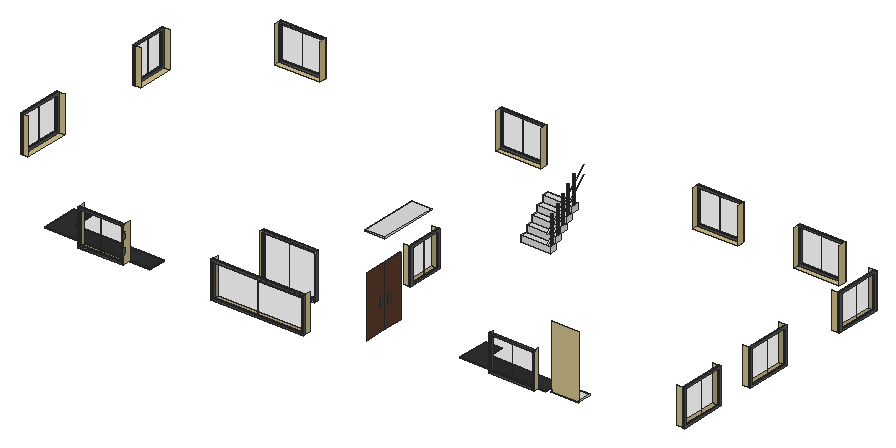
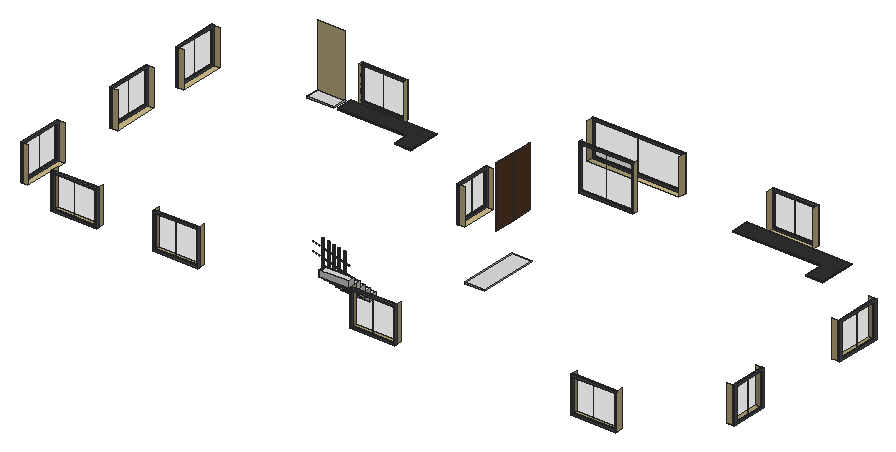
# SketchUp Ruby script. Lengths in inches.
U = 1.inch
M = Sketchup.active_model
def pt(a) = Geom::Point3d.new(a.map { |v| v * U })
def face(e, loops, mat)
  f = e.add_face(loops[0].map { |a| pt(a) })
  loops[1..].each { |l| e.add_face(l.map { |a| pt(a) }).erase! }
  f.material = f.back_material = mat if mat
  f
end
# faces: each face lists its corners as indices into pts; further lists are holes
def faces(e, pts, list, mat = nil) = list.each { |f| face(e, (f[0].is_a?(Array) ? f : [f]).map { |l| l.map { |i| pts[i] } }, mat) }
# xy, xz, yz: faces in a plane at the given z, y or x. An outline is a flat list of corners, or four numbers for a rectangle; further outlines are holes
def ring(l) = l.size == 4 ? [[l[0], l[1]], [l[2], l[1]], [l[2], l[3]], [l[0], l[3]]] : l.each_slice(2).to_a
def flat(e, list, mat, &to3) = list.each { |f| face(e, (f[0].is_a?(Array) ? f : [f]).map { |l| ring(l).map { |u, v| to3.(u, v) } }, mat) }
def xy(e, z, list, mat = nil) = flat(e, list, mat) { |x, y| [x, y, z] }
def xz(e, y, list, mat = nil) = flat(e, list, mat) { |x, z| [x, y, z] }
def yz(e, x, list, mat = nil) = flat(e, list, mat) { |y, z| [x, y, z] }
def lines(e, pts, list) = list.each { |a, b| e.add_line(pt(pts[a]), pt(pts[b])) }
# prism: a flat outline (further loops are holes) pulled along v
def prism(e, loops, v, mat = nil)
  f = face(e, loops, mat); d = Geom::Vector3d.new(v.map { |x| x * U })
  f.pushpull(f.normal.samedirection?(d) ? d.length : -d.length)
end
def box(e, o, s, mat = nil) = prism(e, [[o, [o[0] + s[0], o[1], o[2]], [o[0] + s[0], o[1] + s[1], o[2]], [o[0], o[1] + s[1], o[2]]]], [0, 0, s[2]], mat)
def at(x, y, z, deg = 0) = Geom::Transformation.translation(pt([x, y, z])) * Geom::Transformation.rotation(ORIGIN, Z_AXIS, deg.degrees)
def axes(o, x, y, z) = Geom::Transformation.new([*x, 0, *y, 0, *z, 0, *pt(o).to_a, 1])
def part(name) = M.definitions.add(name)
# library, detail: a bought-in or finely detailed component or shape, given as its bounding box
def library(name, o, s) = part(name).tap { |d| box(d.entities, o, s) }
def detail(e, o, s) = box(e.add_group.entities, o, s)
def put(e, d, t, mat = nil) = e.add_instance(d, t).tap { |i| i.material = mat if mat }
def group(e, t, mat = nil) = e.add_group.tap { |g| g.transformation = t; g.material = mat if mat }.entities
root = M.entities
M.materials.add("Flooring Laminate Dark Smoked 375cm").color = [91, 60, 43]
M.materials.add("Glass Smoked Distorted 001").color = [38, 38, 38]
M.materials["Glass Smoked Distorted 001"].alpha = 0.1
M.materials.add("Granite Black Pearl 150cm").color = [48, 48, 48]
M.materials.add("Marble White SSS 100cm").color = [222, 222, 222]
M.materials.add("Metal Sandblasted Black 200cm").color = [86, 90, 95]
M.materials.add("Wall Paint Fine Grain 01 Yellow 100cm").color = [207, 190, 139]
c1 = part("Group\#124")
p = [[0,61.03,56],[0.26,0,0],[0.46,0,0],[0.2,61.03,56]]
faces(c1.entities,p,[[0,1,2,3]])
c2 = part("Group\#8")
box(c2.entities,[0,0,0],[59.16,0.31,44])
c3 = part("Group\#10")
box(c3.entities,[0,-0.31,0],[34,0.31,56])
c4 = part("Group\#41")
box(c4.entities,[-0.31,0,0],[0.31,22,44])
c5 = part("Group\#43")
box(c5.entities,[0,-0.31,0],[28,0.31,44])
c6 = part("Group\#49")
box(c6.entities,[0,-0.25,0],[28,0.25,44])
c7 = part("Group\#51")
box(c7.entities,[0,0,0],[0.31,22,44])
c8 = part("Group\#55")
box(c8.entities,[0,0,0],[0.31,28,44])
c9 = part("Group\#61")
box(c9.entities,[-0.31,0,0],[0.31,28,44])
c10 = part("Group\#63")
box(c10.entities,[-0.31,0,0],[0.31,28,44])
c11 = part("Group\#65")
box(c11.entities,[-0.31,0,0],[0.31,28,44])
c12 = part("Group\#67")
box(c12.entities,[0,-0.31,0],[28,0.31,44])
c13 = part("Group\#71")
box(c13.entities,[0,-0.31,0],[28,0.31,44])
c14 = part("Group\#75")
box(c14.entities,[0,0,0],[28,0.31,44])
c15 = part("Group\#57")
box(c15.entities,[0,0,0],[28,0.31,44])
xy(root,36,[[170.63,1.5,230.63,10.5],[347.5,1.5,469.81,10.5],[669.19,60,729.19,64.5],[363.31,61.5,435.31,66],[744.31,67.6875,780.31,69],
  [889.81,94,898.81,154],[1.81,117.625,10.81,177.625],[481.81,150.6875,490.81,198.6875],[889.81,203.625,898.81,263.625],[1.81,303.6875,10.81,351.6875],
  [889.81,351.6875,898.81,411.6875],[88.19,429,148.19,437.875],[381.31,429,441.31,437.875],[642.44,429,702.44,438],[777,429,837,438]],"Wall Paint Fine Grain 01 Yellow 100cm")
xz(root,69,[[744.31,36,780.31,120]],"Wall Paint Fine Grain 01 Yellow 100cm")
xz(root,94,[[889.81,36,898.81,84]],"Wall Paint Fine Grain 01 Yellow 100cm")
xz(root,117.625,[[1.81,36,10.81,84]],"Wall Paint Fine Grain 01 Yellow 100cm")
xz(root,150.6875,[[481.81,36,490.81,84]],"Wall Paint Fine Grain 01 Yellow 100cm")
xz(root,154,[[889.81,36,898.81,84]],"Wall Paint Fine Grain 01 Yellow 100cm")
xz(root,177.625,[[1.81,36,10.81,84]],"Wall Paint Fine Grain 01 Yellow 100cm")
xz(root,198.6875,[[481.81,36,490.81,84]],"Wall Paint Fine Grain 01 Yellow 100cm")
xz(root,203.625,[[889.81,36,898.81,84]],"Wall Paint Fine Grain 01 Yellow 100cm")
xz(root,263.625,[[889.81,36,898.81,84]],"Wall Paint Fine Grain 01 Yellow 100cm")
xz(root,303.6875,[[1.81,36,10.81,84]],"Wall Paint Fine Grain 01 Yellow 100cm")
xz(root,351.6875,[[1.81,36,10.81,84],[889.81,36,898.81,84]],"Wall Paint Fine Grain 01 Yellow 100cm")
xz(root,411.6875,[[889.81,36,898.81,84]],"Wall Paint Fine Grain 01 Yellow 100cm")
yz(root,88.19,[[429,36,437.875,84]],"Wall Paint Fine Grain 01 Yellow 100cm")
yz(root,148.19,[[429,36,437.875,84]],"Wall Paint Fine Grain 01 Yellow 100cm")
yz(root,170.63,[[1.5,36,10.5,84]],"Wall Paint Fine Grain 01 Yellow 100cm")
yz(root,230.63,[[1.5,36,10.5,84]],"Wall Paint Fine Grain 01 Yellow 100cm")
yz(root,347.5,[[1.5,36,10.5,84]],"Wall Paint Fine Grain 01 Yellow 100cm")
yz(root,363.31,[[61.5,36,66,96]],"Wall Paint Fine Grain 01 Yellow 100cm")
yz(root,381.31,[[429,36,437.875,84]],"Wall Paint Fine Grain 01 Yellow 100cm")
yz(root,435.31,[[61.5,36,66,96]],"Wall Paint Fine Grain 01 Yellow 100cm")
yz(root,441.31,[[429,36,437.875,84]],"Wall Paint Fine Grain 01 Yellow 100cm")
yz(root,469.81,[[1.5,36,10.5,84]],"Wall Paint Fine Grain 01 Yellow 100cm")
yz(root,642.44,[[429,36,438,84]],"Wall Paint Fine Grain 01 Yellow 100cm")
yz(root,669.19,[[60,36,64.5,84]],"Wall Paint Fine Grain 01 Yellow 100cm")
yz(root,702.44,[[429,36,438,84]],"Wall Paint Fine Grain 01 Yellow 100cm")
yz(root,729.19,[[60,36,64.5,84]],"Wall Paint Fine Grain 01 Yellow 100cm")
yz(root,777,[[429,36,438,84]],"Wall Paint Fine Grain 01 Yellow 100cm")
yz(root,837,[[429,36,438,84]],"Wall Paint Fine Grain 01 Yellow 100cm")
g1 = group(root,at(489.5,80.6875,2),"Flooring Laminate Dark Smoked 375cm")
xy(g1,0,[[-0.71,0,0,28]])
xy(g1,80,[[-0.71,0,0,28]])
xz(g1,0,[[-0.71,0,0,80]],"Flooring Laminate Dark Smoked 375cm")
xz(g1,28,[[-0.71,0,0,80]],"Flooring Laminate Dark Smoked 375cm")
yz(g1,-0.71,[[0,0,28,80]],"Flooring Laminate Dark Smoked 375cm")
yz(g1,0,[[0,0,28,80]],"Flooring Laminate Dark Smoked 375cm")
g2 = group(root,at(489.5,108.6875,2),"Flooring Laminate Dark Smoked 375cm")
xy(g2,0,[[-0.71,0,0,28]])
xy(g2,80,[[-0.71,0,0,28]])
xz(g2,0,[[-0.71,0,0,80]],"Flooring Laminate Dark Smoked 375cm")
xz(g2,28,[[-0.71,0,0,80]],"Flooring Laminate Dark Smoked 375cm")
yz(g2,-0.71,[[0,0,28,80]],"Flooring Laminate Dark Smoked 375cm")
yz(g2,0,[[0,0,28,80]],"Flooring Laminate Dark Smoked 375cm")
g3 = group(root,at(490.81,334.5,8))
box(g3,[0,0,0],[39,9,8],"Marble White SSS 100cm")
g4 = group(g3,at(36.5,3.5,8),"Metal Sandblasted Black 200cm")
xy(g4,0,[[1,0,0.74,0.03,0.5,0.13,0.29,0.29,0.13,0.5,0.03,0.74,0,1,0.03,1.26,0.13,1.5,0.29,1.71,0.5,1.87,0.74,1.97,1,2,1.26,1.97,1.5,1.87,1.71,1.71,1.87,1.5,1.97,1.26,2,1,1.97,0.74,1.87,0.5,1.71,0.29,1.5,0.13,1.26,0.03]])
xy(g4,36,[[1,0,1.26,0.03,1.5,0.13,1.71,0.29,1.87,0.5,1.97,0.74,2,1,1.97,1.26,1.87,1.5,1.71,1.71,1.5,1.87,1.26,1.97,1,2,0.74,1.97,0.5,1.87,0.29,1.71,0.13,1.5,0.03,1.26,0,1,0.03,0.74,0.13,0.5,0.29,0.29,0.5,0.13,0.74,0.03]])
p = [[0.5,0.13,0],[0.74,0.03,0],[0.74,0.03,36],[0.5,0.13,36],[1,0,0],[1,0,36],
  [1.26,0.03,0],[1.26,0.03,36],[1.5,0.13,0],[1.5,0.13,36],[0.29,0.29,0],[0.29,0.29,36],
  [1.71,0.29,0],[1.71,0.29,36],[0.13,0.5,0],[0.13,0.5,36],[1.87,0.5,0],[1.87,0.5,36],
  [0.03,0.74,0],[0.03,0.74,36],[1.97,0.74,0],[1.97,0.74,36],[0,1,0],[0,1,36],
  [2,1,0],[2,1,36],[0.03,1.26,0],[0.03,1.26,36],[1.97,1.26,0],[1.97,1.26,36],
  [0.13,1.5,0],[0.13,1.5,36],[1.87,1.5,0],[1.87,1.5,36],[0.29,1.71,0],[0.29,1.71,36],
  [1.71,1.71,0],[1.71,1.71,36],[0.5,1.87,0],[0.5,1.87,36],[1.5,1.87,0],[1.5,1.87,36],
  [0.74,1.97,0],[0.74,1.97,36],[1.26,1.97,0],[1.26,1.97,36],[1,2,0],[1,2,36]]
faces(g4,p,[[0,1,2,3],[1,4,5,2],[4,6,7,5],[6,8,9,7],[10,0,3,11],[8,12,13,9],[14,10,11,15],[12,16,17,13],
  [18,14,15,19],[16,20,21,17],[22,18,19,23],[20,24,25,21],[26,22,23,27],[24,28,29,25],[30,26,27,31],[28,32,33,29],
  [34,30,31,35],[32,36,37,33],[38,34,35,39],[36,40,41,37],[42,38,39,43],[40,44,45,41],[46,42,43,47],[44,46,47,45]],"Metal Sandblasted Black 200cm")
g5 = group(root,at(490.81,343.5,16))
box(g5,[0,0,0],[39,9,8],"Marble White SSS 100cm")
g6 = group(g5,at(36.5,3.5,8),"Metal Sandblasted Black 200cm")
xy(g6,0,[[1,0,0.74,0.03,0.5,0.13,0.29,0.29,0.13,0.5,0.03,0.74,0,1,0.03,1.26,0.13,1.5,0.29,1.71,0.5,1.87,0.74,1.97,1,2,1.26,1.97,1.5,1.87,1.71,1.71,1.87,1.5,1.97,1.26,2,1,1.97,0.74,1.87,0.5,1.71,0.29,1.5,0.13,1.26,0.03]])
xy(g6,36,[[1,0,1.26,0.03,1.5,0.13,1.71,0.29,1.87,0.5,1.97,0.74,2,1,1.97,1.26,1.87,1.5,1.71,1.71,1.5,1.87,1.26,1.97,1,2,0.74,1.97,0.5,1.87,0.29,1.71,0.13,1.5,0.03,1.26,0,1,0.03,0.74,0.13,0.5,0.29,0.29,0.5,0.13,0.74,0.03]])
p = [[0.5,0.13,0],[0.74,0.03,0],[0.74,0.03,36],[0.5,0.13,36],[1,0,0],[1,0,36],
  [1.26,0.03,0],[1.26,0.03,36],[1.5,0.13,0],[1.5,0.13,36],[0.29,0.29,0],[0.29,0.29,36],
  [1.71,0.29,0],[1.71,0.29,36],[0.13,0.5,0],[0.13,0.5,36],[1.87,0.5,0],[1.87,0.5,36],
  [0.03,0.74,0],[0.03,0.74,36],[1.97,0.74,0],[1.97,0.74,36],[0,1,0],[0,1,36],
  [2,1,0],[2,1,36],[0.03,1.26,0],[0.03,1.26,36],[1.97,1.26,0],[1.97,1.26,36],
  [0.13,1.5,0],[0.13,1.5,36],[1.87,1.5,0],[1.87,1.5,36],[0.29,1.71,0],[0.29,1.71,36],
  [1.71,1.71,0],[1.71,1.71,36],[0.5,1.87,0],[0.5,1.87,36],[1.5,1.87,0],[1.5,1.87,36],
  [0.74,1.97,0],[0.74,1.97,36],[1.26,1.97,0],[1.26,1.97,36],[1,2,0],[1,2,36]]
faces(g6,p,[[0,1,2,3],[1,4,5,2],[4,6,7,5],[6,8,9,7],[10,0,3,11],[8,12,13,9],[14,10,11,15],[12,16,17,13],
  [18,14,15,19],[16,20,21,17],[22,18,19,23],[20,24,25,21],[26,22,23,27],[24,28,29,25],[30,26,27,31],[28,32,33,29],
  [34,30,31,35],[32,36,37,33],[38,34,35,39],[36,40,41,37],[42,38,39,43],[40,44,45,41],[46,42,43,47],[44,46,47,45]],"Metal Sandblasted Black 200cm")
put(root,c1,at(528.11,331,20))
g7 = group(root,at(490.81,352.5,24))
box(g7,[0,0,0],[39,9,8],"Marble White SSS 100cm")
g8 = group(g7,at(36.5,3.5,8),"Metal Sandblasted Black 200cm")
prism(g8,[[[1.71,1.71,0],[1.87,1.5,0],[1.97,1.26,0],[2,1,0],[1.97,0.74,0],[1.87,0.5,0],[1.71,0.29,0],[1.5,0.13,0],[1.26,0.03,0],[1,0,0],[0.74,0.03,0],[0.5,0.13,0],[0.29,0.29,0],[0.13,0.5,0],[0.03,0.74,0],[0,1,0],[0.03,1.26,0],[0.13,1.5,0],[0.29,1.71,0],[0.5,1.87,0],[0.74,1.97,0],[1,2,0],[1.26,1.97,0],[1.5,1.87,0]]],[0,0,36])
g9 = group(root,at(490.81,361.5,32))
box(g9,[0,0,0],[39,9,8],"Marble White SSS 100cm")
g10 = group(g9,at(36.5,3.5,8),"Metal Sandblasted Black 200cm")
xy(g10,0,[[1,0,0.74,0.03,0.5,0.13,0.29,0.29,0.13,0.5,0.03,0.74,0,1,0.03,1.26,0.13,1.5,0.29,1.71,0.5,1.87,0.74,1.97,1,2,1.26,1.97,1.5,1.87,1.71,1.71,1.87,1.5,1.97,1.26,2,1,1.97,0.74,1.87,0.5,1.71,0.29,1.5,0.13,1.26,0.03]])
xy(g10,36,[[1,0,1.26,0.03,1.5,0.13,1.71,0.29,1.87,0.5,1.97,0.74,2,1,1.97,1.26,1.87,1.5,1.71,1.71,1.5,1.87,1.26,1.97,1,2,0.74,1.97,0.5,1.87,0.29,1.71,0.13,1.5,0.03,1.26,0,1,0.03,0.74,0.13,0.5,0.29,0.29,0.5,0.13,0.74,0.03]])
p = [[0.5,0.13,0],[0.74,0.03,0],[0.74,0.03,36],[0.5,0.13,36],[1,0,0],[1,0,36],
  [1.26,0.03,0],[1.26,0.03,36],[1.5,0.13,0],[1.5,0.13,36],[0.29,0.29,0],[0.29,0.29,36],
  [1.71,0.29,0],[1.71,0.29,36],[0.13,0.5,0],[0.13,0.5,36],[1.87,0.5,0],[1.87,0.5,36],
  [0.03,0.74,0],[0.03,0.74,36],[1.97,0.74,0],[1.97,0.74,36],[0,1,0],[0,1,36],
  [2,1,0],[2,1,36],[0.03,1.26,0],[0.03,1.26,36],[1.97,1.26,0],[1.97,1.26,36],
  [0.13,1.5,0],[0.13,1.5,36],[1.87,1.5,0],[1.87,1.5,36],[0.29,1.71,0],[0.29,1.71,36],
  [1.71,1.71,0],[1.71,1.71,36],[0.5,1.87,0],[0.5,1.87,36],[1.5,1.87,0],[1.5,1.87,36],
  [0.74,1.97,0],[0.74,1.97,36],[1.26,1.97,0],[1.26,1.97,36],[1,2,0],[1,2,36]]
faces(g10,p,[[0,1,2,3],[1,4,5,2],[4,6,7,5],[6,8,9,7],[10,0,3,11],[8,12,13,9],[14,10,11,15],[12,16,17,13],
  [18,14,15,19],[16,20,21,17],[22,18,19,23],[20,24,25,21],[26,22,23,27],[24,28,29,25],[30,26,27,31],[28,32,33,29],
  [34,30,31,35],[32,36,37,33],[38,34,35,39],[36,40,41,37],[42,38,39,43],[40,44,45,41],[46,42,43,47],[44,46,47,45]],"Metal Sandblasted Black 200cm")
put(root,c1,at(528.11,331,32))
g11 = group(root,at(490.81,114.56,34),"Metal Sandblasted Black 200cm")
box(g11,[0,0,0],[0.5,1.49,8])
g12 = group(root,at(490.81,101.29,34),"Metal Sandblasted Black 200cm")
box(g12,[0,0,0],[0.5,1.42,8])
g13 = group(root,at(347.5,1.5,36))
prism(g13,[[[0,-1.5,0],[122.3125,-1.5,0],[122.3125,-1.5,48],[0,-1.5,48]],[[120.3125,-1.5,2],[2,-1.5,2],[2,-1.5,46],[120.3125,-1.5,46]]],[0,3,0],"Metal Sandblasted Black 200cm")
put(g13,c2,at(2,-0.0625,2),"Glass Smoked Distorted 001")
put(g13,c2,at(61.16,-0.38,2),"Glass Smoked Distorted 001")
g14 = group(root,at(363.31,66,36))
prism(g14,[[[72,1.5,0],[0,1.5,0],[0,1.5,60],[72,1.5,60]],[[2,1.5,2],[70,1.5,2],[70,1.5,58],[2,1.5,58]]],[0,-3,0],"Metal Sandblasted Black 200cm")
put(g14,c3,at(36,-0.125,2),"Glass Smoked Distorted 001")
put(g14,c3,at(2,0.19,2),"Glass Smoked Distorted 001")
g15 = group(root,at(490.81,150.6875,36))
prism(g15,[[[1.5,0,0],[1.5,48,0],[1.5,48,48],[1.5,0,48]],[[1.5,2,2],[1.5,2,46],[1.5,46,46],[1.5,46,2]]],[-3,0,0],"Metal Sandblasted Black 200cm")
put(g15,c4,at(-0.1875,2,2),"Glass Smoked Distorted 001")
put(g15,c4,at(0.13,24,2),"Glass Smoked Distorted 001")
g16 = group(root,at(381.31,438,36))
prism(g16,[[[60,1.5,0],[0,1.5,0],[0,1.5,48],[60,1.5,48]],[[2,1.5,46],[2,1.5,2],[58,1.5,2],[58,1.5,46]]],[0,-3,0],"Metal Sandblasted Black 200cm")
put(g16,c5,at(30,-0.125,2),"Glass Smoked Distorted 001")
put(g16,c5,at(2,0.19,2),"Glass Smoked Distorted 001")
g17 = group(root,at(88.19,438,36))
prism(g17,[[[60,1.5,0],[0,1.5,0],[0,1.5,48],[60,1.5,48]],[[2,1.5,2],[58,1.5,2],[58,1.5,46],[2,1.5,46]]],[0,-3,0],"Metal Sandblasted Black 200cm")
put(g17,c6,at(30,0.0625,2),"Glass Smoked Distorted 001")
put(g17,c6,at(2,0.3125,2),"Glass Smoked Distorted 001")
g18 = group(root,at(1.81,303.6875,36))
prism(g18,[[[-1.5,48,0],[-1.5,0,0],[-1.5,0,48],[-1.5,48,48]],[[-1.5,2,46],[-1.5,2,2],[-1.5,46,2],[-1.5,46,46]]],[3,0,0],"Metal Sandblasted Black 200cm")
put(g18,c7,at(-0.0625,24,2),"Glass Smoked Distorted 001")
put(g18,c7,at(-0.38,2,2),"Glass Smoked Distorted 001")
g19 = group(root,at(1.81,117.625,36))
prism(g19,[[[-1.5,60,0],[-1.5,0,0],[-1.5,0,48],[-1.5,60,48]],[[-1.5,58,46],[-1.5,2,46],[-1.5,2,2],[-1.5,58,2]]],[3,0,0],"Metal Sandblasted Black 200cm")
put(g19,c8,at(-0.25,30,2),"Glass Smoked Distorted 001")
put(g19,c8,at(-0.56,2,2),"Glass Smoked Distorted 001")
g20 = group(root,at(898.81,94,36))
prism(g20,[[[1.5,60,0],[1.5,60,48],[1.5,0,48],[1.5,0,0]],[[1.5,58,46],[1.5,58,2],[1.5,2,2],[1.5,2,46]]],[-3,0,0],"Metal Sandblasted Black 200cm")
put(g20,c9,at(0,2,2),"Glass Smoked Distorted 001")
put(g20,c9,at(0.31,30,2),"Glass Smoked Distorted 001")
g21 = group(root,at(898.81,203.625,36))
prism(g21,[[[1.5,0,0],[1.5,60,0],[1.5,60,48],[1.5,0,48]],[[1.5,58,2],[1.5,2,2],[1.5,2,46],[1.5,58,46]]],[-3,0,0],"Metal Sandblasted Black 200cm")
put(g21,c10,at(-0.0625,2,2),"Glass Smoked Distorted 001")
put(g21,c10,at(0.25,30,2),"Glass Smoked Distorted 001")
g22 = group(root,at(898.81,351.6875,36))
prism(g22,[[[1.5,0,0],[1.5,60,0],[1.5,60,48],[1.5,0,48]],[[1.5,58,46],[1.5,58,2],[1.5,2,2],[1.5,2,46]]],[-3,0,0],"Metal Sandblasted Black 200cm")
put(g22,c11,at(-0.1875,2,2),"Glass Smoked Distorted 001")
put(g22,c11,at(0.13,30,2),"Glass Smoked Distorted 001")
g23 = group(root,at(777,438,36))
prism(g23,[[[60,1.5,0],[0,1.5,0],[0,1.5,48],[60,1.5,48]],[[2,1.5,46],[2,1.5,2],[58,1.5,2],[58,1.5,46]]],[0,-3,0],"Metal Sandblasted Black 200cm")
put(g23,c12,at(30,0.0625,2),"Glass Smoked Distorted 001")
put(g23,c12,at(2,0.38,2),"Glass Smoked Distorted 001")
g24 = group(root,at(642.44,438,36))
prism(g24,[[[60,1.5,0],[0,1.5,0],[0,1.5,48],[60,1.5,48]],[[2,1.5,46],[2,1.5,2],[58,1.5,2],[58,1.5,46]]],[0,-3,0],"Metal Sandblasted Black 200cm")
put(g24,c13,at(30,-0.0625,2),"Glass Smoked Distorted 001")
put(g24,c13,at(2,0.25,2),"Glass Smoked Distorted 001")
g25 = group(root,at(669.19,60,36))
prism(g25,[[[0,-1.5,0],[60,-1.5,0],[60,-1.5,48],[0,-1.5,48]],[[58,-1.5,46],[58,-1.5,2],[2,-1.5,2],[2,-1.5,46]]],[0,3,0],"Metal Sandblasted Black 200cm")
put(g25,c14,at(2,0.3125,2),"Glass Smoked Distorted 001")
put(g25,c14,at(30,0,2),"Glass Smoked Distorted 001")
g26 = group(root,at(626.14,64.5,36),"Granite Black Pearl 150cm")
prism(g26,[[[113.67,0,0],[0,0,0],[0,42,0],[22,42,0],[22,22,0],[113.67,22,0]]],[0,0,1.57],"Granite Black Pearl 150cm")
g27 = group(root,at(744.31,69,36),"Marble White SSS 100cm")
box(g27,[0,0,0],[36,18,1.57],"Marble White SSS 100cm")
g28 = group(root,at(138.81,10.5,36),"Granite Black Pearl 150cm")
prism(g28,[[[-20,0,0],[-20,48,0],[2,48,0],[2,22,0],[119.5,22,0],[119.5,0,0]]],[0,0,1.57],"Granite Black Pearl 150cm")
g29 = group(root,at(382.81,213,36),"Marble White SSS 100cm")
box(g29,[-2,0,0],[26,78,1.57],"Marble White SSS 100cm")
g30 = group(root,at(170.63,1.5,36))
prism(g30,[[[0,-1.5,0],[60,-1.5,0],[60,-1.5,48],[0,-1.5,48]],[[58,-1.5,46],[58,-1.5,2],[2,-1.5,2],[2,-1.5,46]]],[0,3,0],"Metal Sandblasted Black 200cm")
put(g30,c15,at(2,0,2),"Glass Smoked Distorted 001")
put(g30,c15,at(30,-0.31,2),"Glass Smoked Distorted 001")
g31 = group(root,at(490.81,370.5,40))
box(g31,[0,0,0],[39,9,8],"Marble White SSS 100cm")
g32 = group(g31,at(36.5,3.5,8),"Metal Sandblasted Black 200cm")
xy(g32,0,[[1,0,0.74,0.03,0.5,0.13,0.29,0.29,0.13,0.5,0.03,0.74,0,1,0.03,1.26,0.13,1.5,0.29,1.71,0.5,1.87,0.74,1.97,1,2,1.26,1.97,1.5,1.87,1.71,1.71,1.87,1.5,1.97,1.26,2,1,1.97,0.74,1.87,0.5,1.71,0.29,1.5,0.13,1.26,0.03]])
xy(g32,36,[[1,0,1.26,0.03,1.5,0.13,1.71,0.29,1.87,0.5,1.97,0.74,2,1,1.97,1.26,1.87,1.5,1.71,1.71,1.5,1.87,1.26,1.97,1,2,0.74,1.97,0.5,1.87,0.29,1.71,0.13,1.5,0.03,1.26,0,1,0.03,0.74,0.13,0.5,0.29,0.29,0.5,0.13,0.74,0.03]])
p = [[0.5,0.13,0],[0.74,0.03,0],[0.74,0.03,36],[0.5,0.13,36],[1,0,0],[1,0,36],
  [1.26,0.03,0],[1.26,0.03,36],[1.5,0.13,0],[1.5,0.13,36],[0.29,0.29,0],[0.29,0.29,36],
  [1.71,0.29,0],[1.71,0.29,36],[0.13,0.5,0],[0.13,0.5,36],[1.87,0.5,0],[1.87,0.5,36],
  [0.03,0.74,0],[0.03,0.74,36],[1.97,0.74,0],[1.97,0.74,36],[0,1,0],[0,1,36],
  [2,1,0],[2,1,36],[0.03,1.26,0],[0.03,1.26,36],[1.97,1.26,0],[1.97,1.26,36],
  [0.13,1.5,0],[0.13,1.5,36],[1.87,1.5,0],[1.87,1.5,36],[0.29,1.71,0],[0.29,1.71,36],
  [1.71,1.71,0],[1.71,1.71,36],[0.5,1.87,0],[0.5,1.87,36],[1.5,1.87,0],[1.5,1.87,36],
  [0.74,1.97,0],[0.74,1.97,36],[1.26,1.97,0],[1.26,1.97,36],[1,2,0],[1,2,36]]
faces(g32,p,[[0,1,2,3],[1,4,5,2],[4,6,7,5],[6,8,9,7],[10,0,3,11],[8,12,13,9],[14,10,11,15],[12,16,17,13],
  [18,14,15,19],[16,20,21,17],[22,18,19,23],[20,24,25,21],[26,22,23,27],[24,28,29,25],[30,26,27,31],[28,32,33,29],
  [34,30,31,35],[32,36,37,33],[38,34,35,39],[36,40,41,37],[42,38,39,43],[40,44,45,41],[46,42,43,47],[44,46,47,45]],"Metal Sandblasted Black 200cm")
